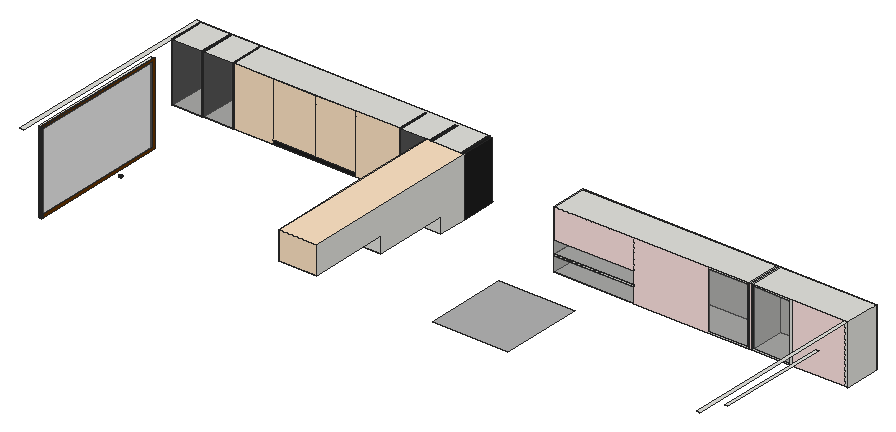
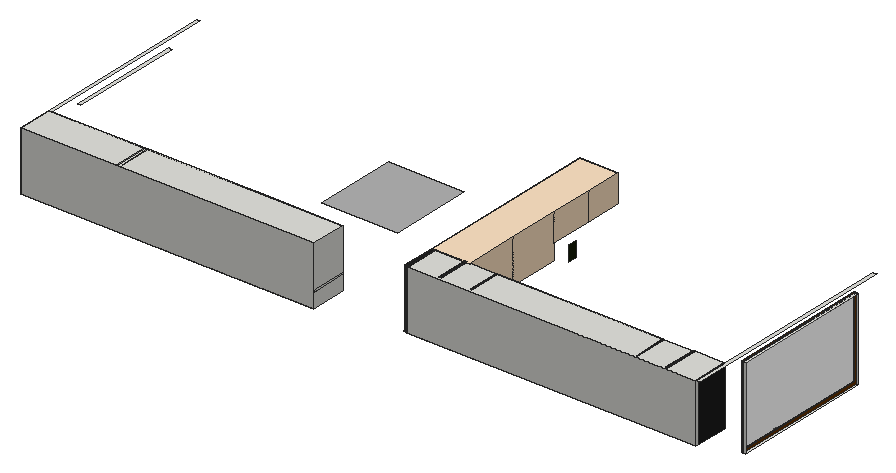
# SketchUp Ruby script. Lengths in inches.
U = 1.inch
M = Sketchup.active_model
def pt(a) = Geom::Point3d.new(a.map { |v| v * U })
def face(e, loops, mat)
  f = e.add_face(loops[0].map { |a| pt(a) })
  loops[1..].each { |l| e.add_face(l.map { |a| pt(a) }).erase! }
  f.material = f.back_material = mat if mat
  f
end
# faces: each face lists its corners as indices into pts; further lists are holes
def faces(e, pts, list, mat = nil) = list.each { |f| face(e, (f[0].is_a?(Array) ? f : [f]).map { |l| l.map { |i| pts[i] } }, mat) }
# xy, xz, yz: faces in a plane at the given z, y or x. An outline is a flat list of corners, or four numbers for a rectangle; further outlines are holes
def ring(l) = l.size == 4 ? [[l[0], l[1]], [l[2], l[1]], [l[2], l[3]], [l[0], l[3]]] : l.each_slice(2).to_a
def flat(e, list, mat, &to3) = list.each { |f| face(e, (f[0].is_a?(Array) ? f : [f]).map { |l| ring(l).map { |u, v| to3.(u, v) } }, mat) }
def xy(e, z, list, mat = nil) = flat(e, list, mat) { |x, y| [x, y, z] }
def xz(e, y, list, mat = nil) = flat(e, list, mat) { |x, z| [x, y, z] }
def yz(e, x, list, mat = nil) = flat(e, list, mat) { |y, z| [x, y, z] }
def lines(e, pts, list) = list.each { |a, b| e.add_line(pt(pts[a]), pt(pts[b])) }
# prism: a flat outline (further loops are holes) pulled along v
def prism(e, loops, v, mat = nil)
  f = face(e, loops, mat); d = Geom::Vector3d.new(v.map { |x| x * U })
  f.pushpull(f.normal.samedirection?(d) ? d.length : -d.length)
end
def box(e, o, s, mat = nil) = prism(e, [[o, [o[0] + s[0], o[1], o[2]], [o[0] + s[0], o[1] + s[1], o[2]], [o[0], o[1] + s[1], o[2]]]], [0, 0, s[2]], mat)
def at(x, y, z, deg = 0) = Geom::Transformation.translation(pt([x, y, z])) * Geom::Transformation.rotation(ORIGIN, Z_AXIS, deg.degrees)
def axes(o, x, y, z) = Geom::Transformation.new([*x, 0, *y, 0, *z, 0, *pt(o).to_a, 1])
def part(name) = M.definitions.add(name)
# library, detail: a bought-in or finely detailed component or shape, given as its bounding box
def library(name, o, s) = part(name).tap { |d| box(d.entities, o, s) }
def detail(e, o, s) = box(e.add_group.entities, o, s)
def put(e, d, t, mat = nil) = e.add_instance(d, t).tap { |i| i.material = mat if mat }
def group(e, t, mat = nil) = e.add_group.tap { |g| g.transformation = t; g.material = mat if mat }.entities
root = M.entities
M.materials.add("[0007_MistyRose]").color = [255, 228, 225]
M.materials.add("[0012_Bisque]").color = [255, 228, 196]
M.materials.add("[Aluminum]").color = [179, 179, 179]
M.materials.add("[Color C08]").color = [102, 51, 0]
M.materials.add("[Color M08]").color = [30, 30, 30]
M.materials.add("[Metal Seamed]").color = [22, 30, 9]
M.materials.add("[Translucent Glass Gray]").color = [128, 128, 128]
M.materials["[Translucent Glass Gray]"].alpha = 0.5
xy(root,47.102,[[0,21.332,3.25,136.27]])
xy(root,61,[[317.619,151,317.619,180,555.119,180,555.119,151,479.26,151,479.26,179.625,476.948,179.625,476.948,151],[476.948,151,479.26,179.625],[555.119,151,557.619,180]])
xy(root,72,[[211,129.67,242.375,153.741],[3.804,153.741,3.804,181.491,3.25,181.491,3.25,182.741,240,182.741,240,181.179,239.274,181.179,239.274,153.741,215.644,153.741,215.644,179.554,213.894,179.554,213.894,153.741,189.956,153.741,189.956,179.491,188.992,179.491,188.992,153.741,53.258,153.741,53.258,180.929,52.706,180.929,52.706,153.741,29.3125,153.741,29.3125,181.116,27.8125,181.116,27.8125,153.741],[240,181.179,242.375,182.741]])
xy(root,72,[[3.25,153.741,3.804,181.491],[27.8125,153.741,29.3125,181.116],[52.706,153.741,53.258,180.929],[188.992,153.741,189.956,179.491],[213.894,153.741,215.644,179.554],
  [239.274,153.741,242.375,181.179]],"[Color M08]")
xy(root,73.375,[[317.619,151,382.931,179.5625]])
xy(root,74.6875,[[317.619,151,382.931,179.5625]])
xy(root,79.3125,[[317.619,26.546,379.119,94.859]],"[Aluminum]")
xy(root,84.656,[[211,68.214,242.375,129.67]])
xy(root,97.3125,[[211,2.741,242.375,68.214]])
xy(root,100.985,[[555.119,28.812,557.619,121.249]])
xy(root,109,[[555.119,0,557.619,151],[317.619,151,476.948,151,476.948,179.625,479.26,179.625,479.26,151,557.619,151,557.619,180,317.619,180],[476.948,151,479.26,179.625]])
xy(root,113.852,[[0,21.332,3.25,136.27]])
xy(root,120,[[0,2.741,3.25,182.741],[3.804,153.741,27.8125,153.741,27.8125,181.116,29.3125,181.116,29.3125,153.741,52.706,153.741,52.706,180.929,53.258,180.929,53.258,153.741,188.992,153.741,188.992,179.491,189.956,179.491,189.956,153.741,213.894,153.741,213.894,179.554,215.644,179.554,215.644,153.741,239.274,153.741,239.274,181.179,240,181.179,240,182.741,3.25,182.741,3.25,181.491,3.804,181.491]])
xy(root,120,[[211,2.741,242.375,153.741]],"[0012_Bisque]")
xy(root,120,[[3.25,153.741,3.804,181.491],[27.8125,153.741,29.3125,181.116],[52.706,153.741,53.258,180.929],[188.992,153.741,189.956,179.491],[213.894,153.741,215.644,179.554],
  [239.274,153.741,242.375,181.179]],"[Color M08]")
xz(root,2.741,[[211,97.3125,242.375,120]],"[0012_Bisque]")
xz(root,21.332,[[0,47.102,3.25,113.852]])
xz(root,68.214,[[211,84.656,242.375,97.3125]])
xz(root,129.67,[[211,72,242.375,84.656]])
xz(root,136.27,[[0,47.102,3.25,113.852]])
xz(root,151,[[[443.198,61,476.948,109],[444.295,62.098,475.85,107.902]],[[479.26,61,511.635,109],[480.358,62.098,510.538,107.902]],[555.119,61,557.619,109],[317.619,73.375,382.931,74.6875]])
xz(root,151,[[382.931,61,443.198,109],[476.948,61,479.26,109],[511.635,61,555.119,109],[317.619,85,382.931,109]],"[0007_MistyRose]")
xz(root,151,[[317.619,61,382.931,73.375],[444.295,62.098,475.85,107.902],[480.358,62.098,510.538,107.902],[317.619,74.6875,382.931,85]],"[Translucent Glass Gray]")
xz(root,153.741,[[53.258,72,85.706,120],[153.456,72,188.992,120],[85.706,74.936,120.269,120],[120.269,74.936,153.456,120]],"[0012_Bisque]")
xz(root,153.741,[[3.25,72,3.804,120],[27.8125,72,29.3125,120],[52.706,72,53.258,120],[85.706,72,153.456,74.936],[188.992,72,189.956,120],
  [213.894,72,215.644,120],[239.274,72,242.375,120]],"[Color M08]")
xz(root,153.741,[[3.804,72,27.8125,120],[29.3125,72,52.706,120],[189.956,72,211,120],[211,72,213.894,120],[215.644,72,239.274,120]],"[Translucent Glass Gray]")
xz(root,179.491,[[188.992,72,189.956,120]],"[Color M08]")
xz(root,179.554,[[213.894,72,215.644,120]],"[Color M08]")
xz(root,179.5625,[[317.619,73.375,382.931,74.6875]])
xz(root,179.625,[[476.948,61,479.26,109]])
xz(root,180,[[317.619,61,557.619,109]])
xz(root,180.929,[[52.706,72,53.258,120]],"[Color M08]")
xz(root,181.116,[[27.8125,72,29.3125,120]],"[Color M08]")
xz(root,181.179,[[239.274,72,240,120],[240,72,242.375,120]],"[Color M08]")
xz(root,181.491,[[3.25,72,3.804,120]],"[Color M08]")
xz(root,182.741,[[3.25,72,240,120]])
yz(root,3.25,[[181.491,72,182.741,120]])
yz(root,3.25,[[153.741,72,181.491,120]],"[Color M08]")
yz(root,3.804,[[153.741,72,181.491,120]],"[Color M08]")
yz(root,27.8125,[[153.741,72,181.116,120]],"[Color M08]")
yz(root,29.3125,[[153.741,72,181.116,120]],"[Color M08]")
yz(root,52.706,[[153.741,72,180.929,120]],"[Color M08]")
yz(root,53.258,[[153.741,72,180.929,120]],"[Color M08]")
yz(root,188.992,[[153.741,72,179.491,120]],"[Color M08]")
yz(root,189.956,[[153.741,72,179.491,120]],"[Color M08]")
yz(root,211,[[129.67,72,129.67,84.656,110.116,84.656,110.116,120,153.741,120,153.741,72],[68.214,84.656,110.116,120],[2.741,97.3125,32.793,120],[32.793,97.3125,68.214,120]],"[0012_Bisque]")
yz(root,211,[[45.786,76.949,53.474,89.387]],"[Metal Seamed]")
yz(root,213.894,[[153.741,72,179.554,120]],"[Color M08]")
yz(root,215.644,[[153.741,72,179.554,120]],"[Color M08]")
yz(root,239.274,[[153.741,72,181.179,120]],"[Color M08]")
yz(root,240,[[181.179,72,182.741,120]])
yz(root,242.375,[[129.67,72,153.741,72,153.741,120,2.741,120,2.741,97.3125,68.214,97.3125,68.214,84.656,129.67,84.656]])
yz(root,242.375,[[153.741,72,181.179,120]],"[Color M08]")
yz(root,317.619,[[151,61,151,73.375,179.5625,73.375,179.5625,74.6875,151,74.6875,151,109,180,109,180,61],[151,73.375,179.5625,74.6875]])
yz(root,382.931,[[151,73.375,179.5625,74.6875]])
yz(root,476.948,[[151,61,179.625,109]])
yz(root,479.26,[[151,61,179.625,109]])
yz(root,557.619,[[151,61,180,109]])
p = [[7.413,98.041,45.233],[7.51,97.855,45.262],[7.558,97.648,45.277],[7.553,97.436,45.275],[7.496,97.233,45.258],[7.39,97.052,45.226],
  [7.243,96.906,45.181],[7.065,96.804,45.127],[6.867,96.754,45.068],[6.664,96.76,45.006],[6.47,96.819,44.947],[6.296,96.93,44.895],
  [6.157,97.084,44.852],[6.059,97.27,44.823],[6.012,97.476,44.809],[6.017,97.688,44.81],[6.074,97.892,44.827],[6.18,98.073,44.859],
  [6.327,98.219,44.904],[6.505,98.32,44.958],[6.702,98.37,45.018],[6.905,98.365,45.079],[7.1,98.305,45.138],[7.273,98.194,45.19],
  [6.13,97.084,44.94],[6.036,97.27,44.899],[5.99,97.476,44.879],[5.995,97.688,44.881],[6.05,97.892,44.905],[6.152,98.073,44.95],
  [6.432,96.819,45.071],[6.265,96.93,44.999],[6.62,96.76,45.153],[5.941,96.93,44.999],[6.02,97.02,44.964],[6.076,97.084,44.94],
  [6.08,97.084,44.946],[5.962,96.93,45.034],[6.081,97.084,44.947],[6.084,97.084,44.951],[5.99,96.93,45.064],[6.245,96.93,45.034],
  [6.127,97.084,44.946],[6.216,96.93,45.064],[6.122,97.084,44.951],[6.054,98.073,44.95],[6.02,98.107,44.964],[5.912,98.219,45.011],
  [5.936,98.219,45.053],[6.06,98.073,44.96],[6.057,98.073,44.954],[6.146,98.073,44.96],[6.27,98.219,45.053],[6.294,98.219,45.011],
  [6.466,98.32,45.086],[5.338,96.754,45.065],[5.55,96.76,45.034],[5.586,96.76,45.153],[5.39,96.754,45.238],[5.754,96.819,45.004],
  [5.774,96.819,45.071],[5.935,96.93,44.977],[5.816,96.819,45.143],[5.873,96.819,45.203],[6.391,96.819,45.143],[6.333,96.819,45.203],
  [6.816,96.754,45.238],[6.09,97.084,44.954],[6.024,96.93,45.086],[6.096,97.084,44.957],[6.0625,96.93,45.1],[6.182,96.93,45.086],
  [6.116,97.084,44.954],[6.144,96.93,45.1],[6.11,97.084,44.957],[6.103,96.93,45.105],[6.103,97.084,44.957],[5.969,98.219,45.088],
  [6.069,98.073,44.969],[5.903,98.219,44.981],[6.01,98.219,45.115],[6.079,98.073,44.976],[6.055,98.219,45.131],[6.091,98.073,44.981],
  [6.138,98.073,44.969],[6.237,98.219,45.088],[6.127,98.073,44.976],[6.197,98.219,45.115],[6.116,98.073,44.981],[6.151,98.219,45.131],
  [6.103,98.219,45.137],[6.103,98.073,44.982],[5.717,98.32,45.009],[5.74,98.32,45.086],[5.786,98.32,45.165],[6.42,98.32,45.165],
  [5.511,98.37,45.04],[5.55,98.37,45.169],[6.657,98.37,45.169],[5.299,98.365,45.071],[5.354,98.365,45.254],[6.852,98.365,45.254],
  [4.946,96.906,45.123],[5.132,96.804,45.096],[5.2,96.804,45.321],[5.028,96.906,45.395],[5.652,96.76,45.266],[5.742,96.76,45.361],
  [5.942,96.819,45.249],[6.021,96.819,45.277],[6.103,96.819,45.287],[6.186,96.819,45.277],[6.264,96.819,45.249],[6.465,96.76,45.361],
  [6.555,96.76,45.266],[7.006,96.804,45.321],[7.178,96.906,45.395],[4.792,97.052,45.146],[4.886,97.052,45.457],[4.682,97.233,45.162],
  [4.784,97.233,45.501],[4.768,98.041,45.15],[4.666,97.855,45.165],[4.77,97.855,45.508],[4.864,98.041,45.467],[4.914,98.194,45.128],
  [4.999,98.194,45.408],[5.095,98.305,45.101],[5.166,98.305,45.335],[5.849,98.32,45.232],[5.926,98.32,45.282],[6.012,98.32,45.313],
  [6.103,98.32,45.324],[6.194,98.32,45.313],[6.357,98.32,45.232],[6.28,98.32,45.282],[7.04,98.305,45.335],[7.207,98.194,45.408],
  [5.62,98.37,45.29],[6.586,98.37,45.29],[5.481,96.754,45.394],[5.315,96.804,45.518],[5.851,96.76,45.432],[5.973,96.76,45.477],
  [6.233,96.76,45.477],[6.356,96.76,45.432],[6.725,96.754,45.394],[6.892,96.804,45.518],[7.32,97.052,45.457],[7.422,97.233,45.501],
  [4.622,97.436,45.171],[4.729,97.436,45.525],[4.616,97.648,45.172],[4.724,97.648,45.528],[7.342,98.041,45.467],[7.436,97.855,45.508],
  [5.716,98.37,45.391],[5.833,98.37,45.468],[6.373,98.37,45.468],[6.49,98.37,45.391],[5.449,98.365,45.417],[6.757,98.365,45.417],
  [5.164,96.906,45.63],[5.605,96.754,45.524],[6.103,96.76,45.492],[6.602,96.754,45.524],[7.042,96.906,45.63],[7.477,97.436,45.525],
  [7.482,97.648,45.528],[5.139,98.194,45.649],[5.285,98.305,45.54],[6.921,98.305,45.54],[7.067,98.194,45.649],[5.964,98.37,45.515],
  [6.103,98.37,45.532],[6.242,98.37,45.515],[5.579,98.365,45.555],[6.627,98.365,45.555],[5.471,96.804,45.684],[5.755,96.754,45.623],
  [5.924,96.754,45.684],[6.282,96.754,45.684],[6.451,96.754,45.623],[6.735,96.804,45.684],[5.041,97.052,45.723],[7.166,97.052,45.723],
  [5.021,98.041,45.738],[7.185,98.041,45.738],[5.448,98.305,45.712],[6.759,98.305,45.712],[5.737,98.365,45.659],[6.469,98.365,45.659],
  [5.351,96.906,45.827],[5.662,96.804,45.809],[6.103,96.754,45.705],[6.544,96.804,45.809],[6.855,96.906,45.827],[4.952,97.233,45.79],
  [7.255,97.233,45.79],[4.903,97.436,45.826],[7.303,97.436,45.826],[4.899,97.648,45.829],[7.307,97.648,45.829],[4.939,97.855,45.799],
  [7.267,97.855,45.799],[5.331,98.194,45.852],[6.876,98.194,45.852],[5.915,98.365,45.723],[6.103,98.365,45.745],[6.291,98.365,45.723],
  [5.877,96.804,45.886],[6.33,96.804,45.886],[5.252,97.052,45.946],[6.954,97.052,45.946],[5.236,98.041,45.965],[6.97,98.041,45.965],
  [5.646,98.305,45.842],[6.561,98.305,45.842],[5.578,96.906,45.976],[6.103,96.804,45.913],[6.628,96.906,45.976],[5.181,97.233,46.031],
  [7.026,97.233,46.031],[5.171,97.855,46.043],[7.036,97.855,46.043],[5.564,98.194,46.005],[6.642,98.194,46.005],[5.868,98.305,45.923],
  [6.103,98.305,45.95],[6.338,98.305,45.923],[5.833,96.906,46.069],[6.373,96.906,46.069],[5.509,97.052,46.115],[6.697,97.052,46.115],
  [5.142,97.436,46.078],[7.064,97.436,46.078],[5.139,97.648,46.082],[7.068,97.648,46.082],[5.826,98.194,46.1],[6.38,98.194,46.1],
  [6.103,96.906,46.1],[5.459,97.233,46.214],[6.747,97.233,46.214],[5.498,98.041,46.136],[6.708,98.041,46.136],[6.103,98.194,46.132],
  [5.798,97.052,46.219],[6.408,97.052,46.219],[5.432,97.436,46.268],[6.774,97.436,46.268],[5.43,97.648,46.273],[5.452,97.855,46.228],
  [6.754,97.855,46.228],[6.777,97.648,46.273],[5.792,98.041,46.243],[6.414,98.041,46.243],[6.103,97.052,46.255],[5.772,97.233,46.328],
  [6.434,97.233,46.328],[5.769,97.855,46.343],[6.4375,97.855,46.343],[6.103,98.041,46.279],[6.103,97.233,46.366],[5.758,97.436,46.386],
  [6.448,97.436,46.386],[5.757,97.648,46.392],[6.449,97.648,46.392],[6.103,97.855,46.382],[6.103,97.436,46.427],[6.103,97.648,46.432],
  [5.356,97.579,45.0625],[5.407,97.579,45.231],[5.495,97.579,45.383],[5.616,97.579,45.511],[5.763,97.579,45.607],[5.928,97.579,45.667],
  [6.103,97.579,45.6875],[6.278,97.579,45.667],[6.443,97.579,45.607],[6.59,97.579,45.511],[6.711,97.579,45.383],[6.8,97.579,45.231],
  [6.851,97.579,45.0625]]
faces(root,p,[[0,1,2,3,4,5,6,7,8,9,10,11,12,13,14,15,16,17,18,19,20,21,22,23],[24,25,13,12],[25,26,14,13],[26,27,15,14],[27,28,16,15],[28,29,17,16],[30,31,11,10],[32,30,10,9],
  [33,34,35,36,37],[37,36,38,39,40],[31,24,12,11],[41,42,24,31],[43,44,42,41],[45,46,47,48,49,50],[51,52,53,29],[29,53,18,17],
  [53,54,19,18],[55,56,57,58],[56,59,60,57],[59,61,33,60],[60,33,37,62],[62,37,40,63],[64,41,31,30],[65,43,41,64],
  [66,32,9,8],[33,61,34],[40,39,67,68],[68,67,69,70],[71,72,44,43],[73,74,72,71],[75,76,74,73],[70,69,76,75],
  [49,48,77,78],[79,47,46],[78,77,80,81],[81,80,82,83],[84,85,52,51],[86,87,85,84],[88,89,87,86],[83,82,90,91],
  [91,90,89,88],[79,92,93,47],[47,93,94,48],[52,95,54,53],[92,96,97,93],[54,98,20,19],[96,99,100,97],[98,101,21,20],
  [102,103,104,105],[103,55,58,104],[57,60,62,106],[106,62,63,107],[63,40,68,108],[108,68,70,109],[109,70,75,110],[111,73,71,112],
  [110,75,73,111],[112,71,43,65],[113,65,64,114],[114,64,30,32],[115,66,8,7],[116,115,7,6],[117,102,105,118],[119,117,118,120],
  [121,122,123,124],[125,121,124,126],[127,125,126,128],[48,94,129,77],[77,129,130,80],[80,130,131,82],[82,131,132,90],[90,132,133,89],
  [85,134,95,52],[87,135,134,85],[89,133,135,87],[136,137,23,22],[99,127,128,100],[93,97,138,94],[95,139,98,54],[101,136,22,21],
  [104,58,140,141],[58,57,106,140],[107,63,108,142],[142,108,109,143],[144,111,112,145],[145,112,65,113],[146,114,32,66],[147,146,66,115],
  [148,116,6,5],[149,148,5,4],[150,119,120,151],[152,150,151,153],[122,152,153,123],[154,155,1,0],[137,154,0,23],[94,138,156,129],
  [129,156,157,130],[135,158,159,134],[134,159,139,95],[97,100,160,138],[139,161,101,98],[105,104,141,162],[140,106,107,163],[143,109,110,164],
  [164,110,111,144],[165,113,114,146],[166,147,115,116],[167,149,4,3],[168,167,3,2],[155,168,2,1],[128,126,169,170],[171,172,137,136],
  [100,128,170,160],[130,157,173,131],[131,173,174,132],[132,174,175,133],[133,175,158,135],[161,171,136,101],[138,160,176,156],[159,177,161,139],
  [141,140,163,178],[163,107,142,179],[179,142,143,180],[181,144,145,182],[182,145,113,165],[183,165,146,147],[118,105,162,184],[185,166,116,148],
  [126,124,186,169],[172,187,154,137],[160,170,188,176],[177,189,171,161],[156,176,190,157],[158,191,177,159],[162,141,178,192],[178,163,179,193],
  [180,143,164,194],[194,164,144,181],[195,182,165,183],[196,183,147,166],[120,118,184,197],[198,185,148,149],[151,120,197,199],[200,198,149,167],
  [153,151,199,201],[202,200,167,168],[123,153,201,203],[204,202,168,155],[124,123,203,186],[187,204,155,154],[170,169,205,188],[189,206,172,171],
  [157,190,207,173],[173,207,208,174],[174,208,209,175],[175,209,191,158],[193,179,180,210],[211,181,182,195],[184,162,192,212],[213,196,166,185],
  [169,186,214,205],[206,215,187,172],[176,188,216,190],[191,217,189,177],[192,178,193,218],[210,180,194,219],[219,194,181,211],[220,195,183,196],
  [197,184,212,221],[222,213,185,198],[186,203,223,214],[215,224,204,187],[188,205,225,216],[217,226,206,189],[190,216,227,207],[207,227,228,208],
  [208,228,229,209],[209,229,217,191],[218,193,210,230],[231,211,195,220],[212,192,218,232],[233,220,196,213],[199,197,221,234],[235,222,198,200],
  [201,199,234,236],[237,235,200,202],[203,201,236,223],[224,237,202,204],[216,225,238,227],[229,239,226,217],[230,210,219,240],[240,219,211,231],
  [221,212,232,241],[242,233,213,222],[205,214,243,225],[226,244,215,206],[227,238,245,228],[228,245,239,229],[232,218,230,246],[247,231,220,233],
  [234,221,241,248],[249,242,222,235],[223,236,250,251],[252,253,237,224],[214,223,251,243],[244,252,224,215],[225,243,254,238],[239,255,244,226],
  [246,230,240,256],[256,240,231,247],[241,232,246,257],[258,247,233,242],[236,234,248,250],[253,249,235,237],[243,251,259,254],[255,260,252,244],
  [238,254,261,245],[245,261,255,239],[257,246,256,262],[262,256,247,258],[248,241,257,263],[264,258,242,249],[251,250,265,259],[260,266,253,252],
  [254,259,267,261],[261,267,260,255],[263,257,262,268],[268,262,258,264],[250,248,263,265],[266,264,249,253],[259,265,269,267],[267,269,266,260],
  [265,263,268,269],[269,268,264,266]])
lines(root,p,[[270,271],[271,272],[272,273],[273,274],[274,275],[275,276],[276,277],[277,278],[278,279],[279,280],[280,281],[281,282]])
g1 = group(root,at(2.0625,20.58,47.1))
xy(g1,0,[[0,0,1.03,115.69]],"[Color C08]")
xy(g1,1.74,[[0,1.78,1.03,113.92]],"[Color C08]")
xy(g1,64.87,[[0,1.78,1.03,113.92]],"[Color C08]")
xy(g1,66.61,[[0,0,1.03,115.69]],"[Color C08]")
xz(g1,0,[[0,0,1.03,66.61]],"[Color C08]")
xz(g1,1.78,[[0,1.74,1.03,64.87]],"[Color C08]")
xz(g1,113.92,[[0,1.74,1.03,64.87]],"[Color C08]")
xz(g1,115.69,[[0,0,1.03,66.61]],"[Color C08]")
yz(g1,0,[[[0,0,115.69,66.61],[1.78,1.74,113.92,64.87]]],"[Color C08]")
yz(g1,1.03,[[[0,0,115.69,66.61],[1.78,1.74,113.92,64.87]]],"[Color C08]")
yz(g1,1.03,[[1.78,1.74,113.92,64.87]],"[Translucent Glass Gray]")
